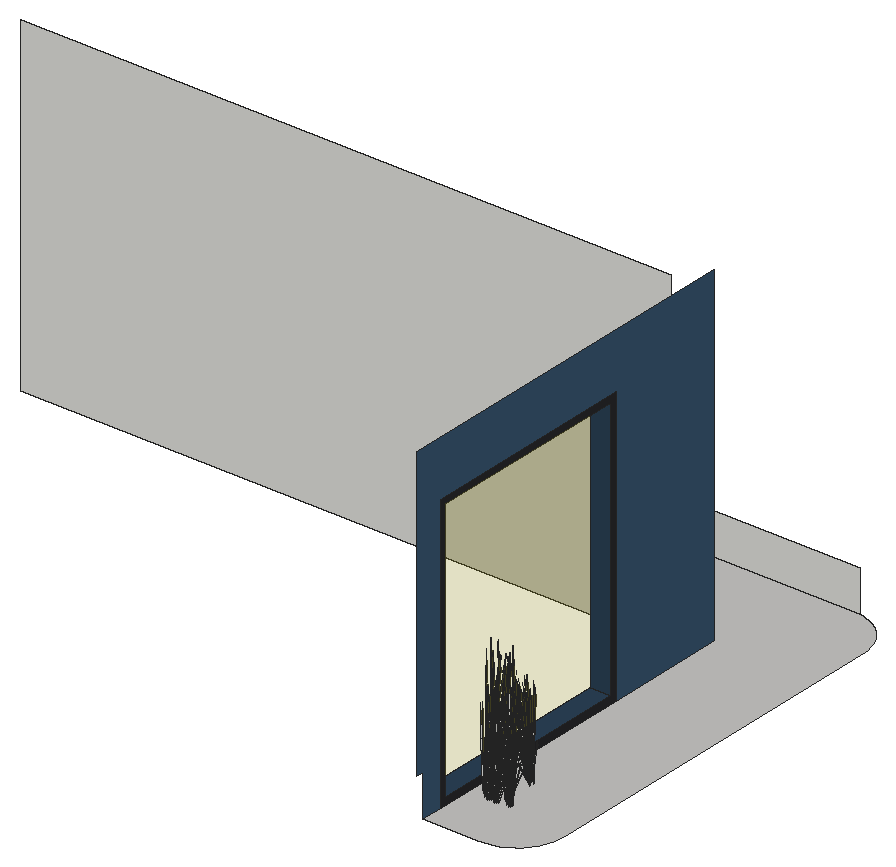
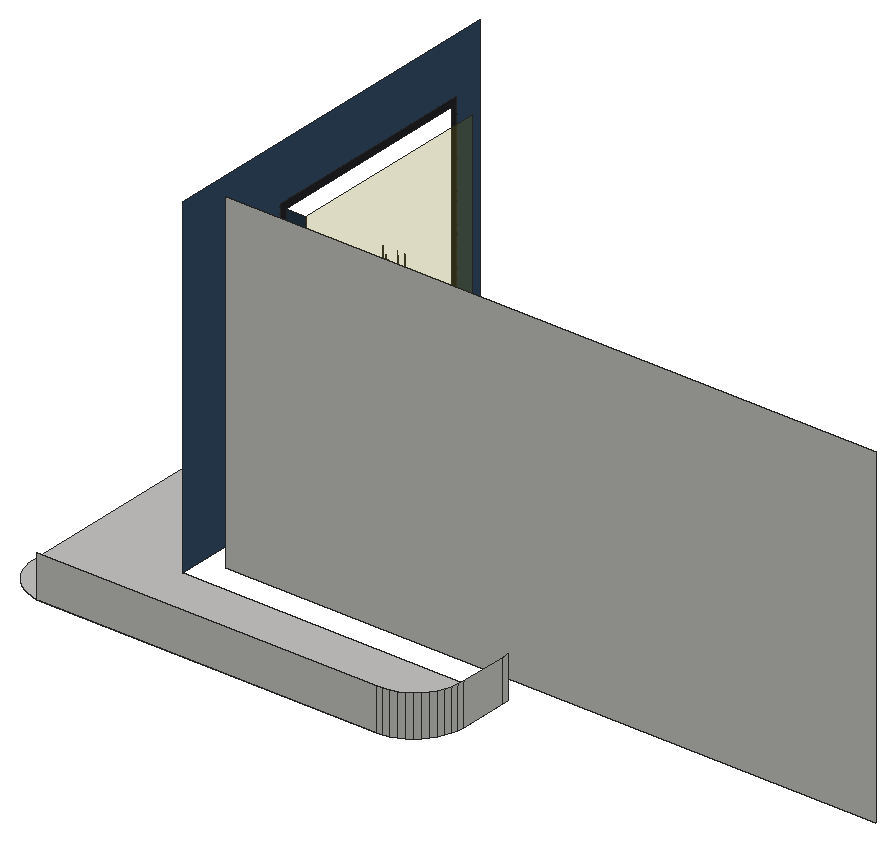
# SketchUp Ruby script. Lengths in inches.
U = 1.inch
M = Sketchup.active_model
def pt(a) = Geom::Point3d.new(a.map { |v| v * U })
def face(e, loops, mat)
  f = e.add_face(loops[0].map { |a| pt(a) })
  loops[1..].each { |l| e.add_face(l.map { |a| pt(a) }).erase! }
  f.material = f.back_material = mat if mat
  f
end
# faces: each face lists its corners as indices into pts; further lists are holes
def faces(e, pts, list, mat = nil) = list.each { |f| face(e, (f[0].is_a?(Array) ? f : [f]).map { |l| l.map { |i| pts[i] } }, mat) }
# xy, xz, yz: faces in a plane at the given z, y or x. An outline is a flat list of corners, or four numbers for a rectangle; further outlines are holes
def ring(l) = l.size == 4 ? [[l[0], l[1]], [l[2], l[1]], [l[2], l[3]], [l[0], l[3]]] : l.each_slice(2).to_a
def flat(e, list, mat, &to3) = list.each { |f| face(e, (f[0].is_a?(Array) ? f : [f]).map { |l| ring(l).map { |u, v| to3.(u, v) } }, mat) }
def xy(e, z, list, mat = nil) = flat(e, list, mat) { |x, y| [x, y, z] }
def xz(e, y, list, mat = nil) = flat(e, list, mat) { |x, z| [x, y, z] }
def yz(e, x, list, mat = nil) = flat(e, list, mat) { |y, z| [x, y, z] }
def lines(e, pts, list) = list.each { |a, b| e.add_line(pt(pts[a]), pt(pts[b])) }
# prism: a flat outline (further loops are holes) pulled along v
def prism(e, loops, v, mat = nil)
  f = face(e, loops, mat); d = Geom::Vector3d.new(v.map { |x| x * U })
  f.pushpull(f.normal.samedirection?(d) ? d.length : -d.length)
end
def box(e, o, s, mat = nil) = prism(e, [[o, [o[0] + s[0], o[1], o[2]], [o[0] + s[0], o[1] + s[1], o[2]], [o[0], o[1] + s[1], o[2]]]], [0, 0, s[2]], mat)
def at(x, y, z, deg = 0) = Geom::Transformation.translation(pt([x, y, z])) * Geom::Transformation.rotation(ORIGIN, Z_AXIS, deg.degrees)
def axes(o, x, y, z) = Geom::Transformation.new([*x, 0, *y, 0, *z, 0, *pt(o).to_a, 1])
def part(name) = M.definitions.add(name)
# library, detail: a bought-in or finely detailed component or shape, given as its bounding box
def library(name, o, s) = part(name).tap { |d| box(d.entities, o, s) }
def detail(e, o, s) = box(e.add_group.entities, o, s)
def put(e, d, t, mat = nil) = e.add_instance(d, t).tap { |i| i.material = mat if mat }
def group(e, t, mat = nil) = e.add_group.tap { |g| g.transformation = t; g.material = mat if mat }.entities
root = M.entities
M.materials.add("Carpet_01_1K").color = [196, 195, 193]
M.materials.add("Carpet_04_1K").color = [56, 85, 112]
M.materials.add("Carpet_04_1K1").color = [43, 65, 85]
M.materials.add("Glass_Basic_01").color = [186, 175, 28]
M.materials["Glass_Basic_01"].alpha = 0.25
M.materials.add("LightPink_Translucent").color = [144, 107, 117]
M.materials["LightPink_Translucent"].alpha = 0.75
M.materials.add("ThomThom - Buttons2").color = [40, 40, 43]
c1 = part("blade")
p = [[2.15,0.21,22],[0,0.17,0],[0.09,0.45,0],[2.18,0.31,22],[2.29,0.31,22],[0.38,0.45,0],
  [2.48,0.24,33],[2.49,0.24,33],[2.48,0.22,33]]
faces(c1.entities,p,[[0,1,2,3],[4,5,2,3],[6,3,4,7],[8,0,3,6]])
c2 = part("seeds")
p = [[0.3,-0.1,1.38],[-0.01,-0.03,1.59],[-0.01,-0.03,0.03],[0.14,-0.07,-0.07],[0.29,-0.03,3],[0.15,0.01,3.11]]
faces(c2.entities,p,[[0,1,2,3],[1,0,4,5]],"LightPink_Translucent")
c3 = part("blade with seeds")
put(c3.entities,c1,at(0,0,0))
put(c3.entities,c2,axes([2.4,0.25,30.99],[1.5799,-0.05474,1.17369],[-0.12525,1.92788,0.29478],[-0.07173,-0.02425,1.56792]))
xy(root,618,[[330.57,640.9,354.57,640.9,357.32,641.08,360.01,641.62,362.61,642.5,365.07,643.71,367.36,645.24,369.42,647.05,371.24,649.12,372.76,651.4,373.98,653.86,374.86,656.47,375.4,659.16,375.57,661.9,375.57,822.84,375.39,825.68,374.85,828.375,373.97,830.97,372.76,833.4375,371.23,835.72,369.42,837.79,367.36,839.6,365.07,841.12,362.61,842.34,360.01,843.22,357.59,843.7,210.57,843.7,207.83,843.52,205.14,842.99,202.54,842.1,200.07,840.89,197.79,839.36,195.73,837.55,193.91,835.48,192.39,833.2,191.17,830.74,190.29,828.14,189.75,825.44,189.57,822.7,189.57,798.7,330.57,798.7]],"Carpet_01_1K")
xy(root,621,[[321.57,652.9,330.57,742.9]],"Carpet_04_1K1")
xz(root,742.9,[[321.57,621,330.57,735]],"Carpet_04_1K1")
xz(root,786.64,[[39.57,618,321.57,762]])
xz(root,843.7,[[210.57,618,357.59,636]])
yz(root,189.57,[[798.7,618,801.7,636],[801.7,618,822.7,636]])
yz(root,321.57,[[652.9,621,742.9,735]],"Glass_Basic_01")
yz(root,330.57,[[640.9,618,649.9,618,649.9,738,745.9,738,745.9,618,798.7,618,798.7,762,637.9,762,637.9,636,640.9,636]],"Carpet_04_1K")
yz(root,330.57,[[[649.9,618,745.9,738],[652.9,621,742.9,735]]],"ThomThom - Buttons2")
p = [[189.57,822.7,618],[189.75,825.44,618],[189.75,825.44,636],[189.57,822.7,636],[190.29,828.14,618],[190.29,828.14,636],
  [191.17,830.74,618],[191.17,830.74,636],[192.39,833.2,618],[192.39,833.2,636],[193.91,835.48,618],[193.91,835.48,636],
  [195.73,837.55,618],[195.73,837.55,636],[197.79,839.36,618],[197.79,839.36,636],[200.07,840.89,618],[200.07,840.89,636],
  [202.54,842.1,618],[202.54,842.1,636],[205.14,842.99,618],[205.14,842.99,636],[207.83,843.52,618],[207.83,843.52,636],
  [210.57,843.7,618],[210.57,843.7,636]]
faces(root,p,[[0,1,2,3],[1,4,5,2],[4,6,7,5],[6,8,9,7],[8,10,11,9],[10,12,13,11],[12,14,15,13],[14,16,17,15],
  [16,18,19,17],[18,20,21,19],[20,22,23,21],[22,24,25,23]])
put(root,c3,axes([342.2,662.9,622.53],[-0.30722,0.06665,-0.35414],[-0.08112,-0.381,0.4572],[-0.08804,0.10234,0.87481]))
put(root,c3,axes([341.27,662.46,620.21],[-0.17124,0.42022,-0.44739],[-0.35581,-0.20224,0.21531],[0,0.09687,1.43643]))
put(root,c3,axes([339.09,662.92,622.53],[-0.30722,0.06665,-0.35414],[-0.08112,-0.381,0.4572],[-0.08804,0.10234,0.87481]))
put(root,c3,axes([350.55,662.74,620.67],[0.04113,0.53214,-0.29095],[-0.42835,0.03218,-0.50002],[-0.07543,0.07088,1.59708]))
put(root,c3,axes([345.11,663.43,622.73],[-0.26024,0.30729,0.48003],[-0.22444,-0.32634,0.3958],[0.1221,0.05668,0.9933]))
put(root,c3,axes([342,663.45,622.73],[-0.26024,0.30729,0.48003],[-0.22444,-0.32634,0.3958],[0.1221,0.05668,0.9933]))
put(root,c3,axes([350.7,662.54,620.21],[-0.17124,0.42022,-0.44739],[-0.35581,-0.20224,0.21531],[0,0.09687,1.43643]))
put(root,c3,axes([348.53,663,622.53],[-0.30722,0.06665,-0.35414],[-0.08112,-0.381,0.4572],[-0.08804,0.10234,0.87481]))
put(root,c3,axes([341.76,663.76,623.65],[0.31145,0.12449,-0.06488],[-0.0958,0.38314,-0.29416],[-0.05094,0.05817,0.97024]))
put(root,c3,axes([343.97,663.05,620.06],[-0.23773,0.35053,-0.62353],[-0.29532,-0.31785,-0.16365],[-0.09526,0.08744,1.37633]))
put(root,c3,axes([338.64,663.78,623.65],[0.31145,0.12449,-0.06488],[-0.0958,0.38314,-0.29416],[-0.05094,0.05817,0.97024]))
put(root,c3,axes([340.85,663.07,620.06],[-0.23773,0.35053,-0.62353],[-0.29532,-0.31785,-0.16365],[-0.09526,0.08744,1.37633]))
put(root,c3,axes([344.28,663.78,623.05],[-0.05451,-0.37564,0.35414],[0.31161,-0.09919,-0.4572],[0.0837,0.10765,0.87481]))
put(root,c3,axes([348.08,663.86,623.65],[0.31145,0.12449,-0.06488],[-0.0958,0.38314,-0.29416],[-0.05094,0.05817,0.97024]))
put(root,c3,axes([350.29,663.15,620.06],[-0.23773,0.35053,-0.62353],[-0.29532,-0.31785,-0.16365],[-0.09526,0.08744,1.37633]))
put(root,c3,axes([341.17,663.8,623.05],[-0.05451,-0.37564,0.35414],[0.31161,-0.09919,-0.4572],[0.0837,0.10765,0.87481]))
put(root,c3,axes([344.39,663.64,620.33],[0.44186,0.15158,0.30756],[-0.11054,0.54181,-0.36492],[-0.07313,0.06781,1.64885]))
put(root,c3,axes([344.36,664.01,620.02],[-0.33032,0.23318,-0.49651],[-0.19744,-0.41812,0],[-0.07523,0.05311,1.57504]))
put(root,c3,axes([341.27,663.66,620.33],[0.44186,0.15158,0.30756],[-0.11054,0.54181,-0.36492],[-0.07313,0.06781,1.64885]))
put(root,c3,axes([345.45,662.625,620.02],[0,0.46636,-0.49651],[-0.39487,0,0],[0,0.10622,1.57504]))
put(root,c3,axes([341.24,664.03,620.02],[-0.33032,0.23318,-0.49651],[-0.19744,-0.41812,0],[-0.07523,0.05311,1.57504]))
put(root,c3,axes([342.34,662.65,620.02],[0,0.46636,-0.49651],[-0.39487,0,0],[0,0.10622,1.57504]))
put(root,c3,axes([344.47,662.68,621.875],[-0.1311,-0.08035,1.71376],[0.27131,-0.33708,0.13857],[0.16909,0.15206,0.73262]))
put(root,c3,axes([341.35,662.7,621.875],[-0.1311,-0.08035,1.71376],[0.27131,-0.33708,0.13857],[0.16909,0.15206,0.73262]))
put(root,c3,axes([350.71,663.74,620.33],[0.44186,0.15158,0.30756],[-0.11054,0.54181,-0.36492],[-0.07313,0.06781,1.64885]))
put(root,c3,axes([344.49,661.62,622.47],[-0.30498,-0.24231,1.38283],[0.32203,-0.37727,0.59665],[0.0984,0.22736,1.33663]))
put(root,c3,axes([350.68,664.11,620.02],[-0.33032,0.23318,-0.49651],[-0.19744,-0.41812,0],[-0.07523,0.05311,1.57504]))
put(root,c3,axes([341.38,661.64,622.47],[-0.30498,-0.24231,1.38283],[0.32203,-0.37727,0.59665],[0.0984,0.22736,1.33663]))
put(root,c3,axes([342.29,662.64,623.03],[0.32648,0.25715,-0.1216],[-0.18809,0.3724,-0.67495],[-0.09224,0.12945,1.02557]))
put(root,c3,axes([339.18,662.66,623.03],[0.32648,0.25715,-0.1216],[-0.18809,0.3724,-0.67495],[-0.09224,0.12945,1.02557]))
put(root,c3,axes([344.95,663.59,620.77],[-0.19872,-0.13409,1.1486],[0.2566,-0.13625,0.84392],[0.06921,0.11541,0.25299]))
put(root,c3,axes([341.84,663.62,620.77],[-0.19872,-0.13409,1.1486],[0.2566,-0.13625,0.84392],[0.06921,0.11541,0.25299]))
put(root,c3,axes([344.25,663.98,623.03],[0.21031,-0.39918,-0.1216],[0.30457,0.22997,-0.67495],[0.10587,0.11278,1.02557]))
put(root,c3,axes([341.14,664,623.03],[0.21031,-0.39918,-0.1216],[0.30457,0.22997,-0.67495],[0.10587,0.11278,1.02557]))
put(root,c3,axes([348.62,662.74,623.03],[0.32648,0.25715,-0.1216],[-0.18809,0.3724,-0.67495],[-0.09224,0.12945,1.02557]))
put(root,c3,axes([342.73,662.53,621.875],[0.08815,-0.14329,1.71376],[0.22258,0.38678,0.13857],[-0.15267,0.17614,0.73262]))
put(root,c3,axes([339.62,662.55,621.875],[0.08815,-0.14329,1.71376],[0.22258,0.38678,0.13857],[-0.15267,0.17614,0.73262]))
put(root,c3,axes([342.46,662.95,622.68],[0.09067,0.42583,-0.51099],[-0.34336,0.07449,-0.3958],[-0.0984,0.11438,0.97773]))
put(root,c3,axes([339.34,662.97,622.68],[0.09067,0.42583,-0.51099],[-0.34336,0.07449,-0.3958],[-0.0984,0.11438,0.97773]))
put(root,c3,axes([349.06,662.63,621.875],[0.08815,-0.14329,1.71376],[0.22258,0.38678,0.13857],[-0.15267,0.17614,0.73262]))
put(root,c3,axes([342.87,663.4375,623.05],[0.23881,-0.24554,0.35414],[0.22606,0.28036,-0.4572],[-0.0344,0.14245,0.87481]))
put(root,c3,axes([344.66,663.93,620.375],[0.22066,0.46731,0],[-0.36918,0.26061,-0.51607],[-0.08408,0.05936,1.63711]))
put(root,c3,axes([339.75,663.46,623.05],[0.23881,-0.24554,0.35414],[0.22606,0.28036,-0.4572],[-0.0344,0.14245,0.87481]))
put(root,c3,axes([348.78,663.05,622.68],[0.09067,0.42583,-0.51099],[-0.34336,0.07449,-0.3958],[-0.0984,0.11438,0.97773]))
put(root,c3,axes([341.54,663.96,620.375],[0.22066,0.46731,0],[-0.36918,0.26061,-0.51607],[-0.08408,0.05936,1.63711]))
put(root,c3,axes([343.98,664.31,622.71],[0.00104,-0.05646,1.77383],[0.30246,-0.2491,-0.16761],[0.10506,0.08891,0.31391]))
put(root,c3,axes([340.87,664.33,622.71],[0.00104,-0.05646,1.77383],[0.30246,-0.2491,-0.16761],[0.10506,0.08891,0.31391]))
put(root,c3,axes([345.01,664.09,619.49],[0.02571,-0.06733,1.76342],[0.32373,-0.19829,-0.26939],[0.09815,0.10263,0.30037]))
put(root,c3,axes([349.19,663.54,623.05],[0.23881,-0.24554,0.35414],[0.22606,0.28036,-0.4572],[-0.0344,0.14245,0.87481]))
put(root,c3,axes([344.47,662.08,620.84],[-0.00964,-0.43909,1.41272],[0.43635,0.11382,0.59816],[-0.1032,0.24027,1.3335]))
put(root,c3,axes([344.58,662.5625,620.09],[0.12941,0.42699,-0.69212],[-0.37279,0.15378,-0.18165],[0.0143,0.14459,1.52773]))
put(root,c3,axes([341.89,664.11,619.49],[0.02571,-0.06733,1.76342],[0.32373,-0.19829,-0.26939],[0.09815,0.10263,0.30037]))
put(root,c3,axes([342.65,663.66,622.73],[-0.29004,-0.02173,0.0643],[0.00795,-0.32812,0.50621],[-0.03035,0.12569,0.77189]))
put(root,c3,axes([350.98,664.03,620.375],[0.22066,0.46731,0],[-0.36918,0.26061,-0.51607],[-0.08408,0.05936,1.63711]))
put(root,c3,axes([341.35,662.11,620.84],[-0.00964,-0.43909,1.41272],[0.43635,0.11382,0.59816],[-0.1032,0.24027,1.3335]))
put(root,c3,axes([341.47,662.58,620.09],[0.12941,0.42699,-0.69212],[-0.37279,0.15378,-0.18165],[0.0143,0.14459,1.52773]))
put(root,c3,axes([339.54,663.68,622.73],[-0.29004,-0.02173,0.0643],[0.00795,-0.32812,0.50621],[-0.03035,0.12569,0.77189]))
put(root,c3,axes([342.04,664.03,619.49],[0.04734,0.04659,1.76342],[0.08027,0.4317,-0.26939],[-0.10492,0.09206,0.30037]))
put(root,c3,axes([342.74,663.69,622.73],[-0.25132,-0.3182,0.48003],[0.2669,-0.27442,0.3958],[-0.04636,0.14929,0.9933]))
put(root,c3,axes([338.92,664.06,619.49],[0.04734,0.04659,1.76342],[0.08027,0.4317,-0.26939],[-0.10492,0.09206,0.30037]))
put(root,c3,axes([344.5,663.78,622.68],[0.34827,-0.11086,-0.51099],[0.06092,0.41983,-0.3958],[0.09354,0.12031,0.97773]))
put(root,c3,axes([339.63,663.71,622.73],[-0.25132,-0.3182,0.48003],[0.2669,-0.27442,0.3958],[-0.04636,0.14929,0.9933]))
put(root,c3,axes([341.39,663.8,622.68],[0.34827,-0.11086,-0.51099],[0.06092,0.41983,-0.3958],[0.09354,0.12031,0.97773]))
put(root,c3,axes([350.79,662.18,620.84],[-0.00964,-0.43909,1.41272],[0.43635,0.11382,0.59816],[-0.1032,0.24027,1.3335]))
put(root,c3,axes([348.98,663.76,622.73],[-0.29004,-0.02173,0.0643],[0.00795,-0.32812,0.50621],[-0.03035,0.12569,0.77189]))
put(root,c3,axes([348.36,664.13,619.49],[0.04734,0.04659,1.76342],[0.08027,0.4317,-0.26939],[-0.10492,0.09206,0.30037]))
put(root,c3,axes([343.54,663.84,623.05],[0.1064,-0.35863,0.35414],[0.31043,0.1046,-0.4572],[0.02846,0.14439,0.87481]))
put(root,c3,axes([349.07,663.79,622.73],[-0.25132,-0.3182,0.48003],[0.2669,-0.27442,0.3958],[-0.04636,0.14929,0.9933]))
put(root,c3,axes([340.42,663.86,623.05],[0.1064,-0.35863,0.35414],[0.31043,0.1046,-0.4572],[0.02846,0.14439,0.87481]))
put(root,c3,axes([349.86,663.94,623.05],[0.1064,-0.35863,0.35414],[0.31043,0.1046,-0.4572],[0.02846,0.14439,0.87481]))
put(root,c3,axes([344.98,664.2,620.67],[-0.22633,-0.01463,1.0506],[0.14947,-0.31064,0.58006],[0.08941,0.11036,0.8241]))
put(root,c3,axes([341.87,664.23,620.67],[-0.22633,-0.01463,1.0506],[0.14947,-0.31064,0.58006],[0.08941,0.11036,0.8241]))
put(root,c3,axes([344.33,664.12,622.73],[-0.16041,0.29625,0.0643],[-0.22843,-0.17248,0.50621],[0.07385,0.09498,0.77189]))
put(root,c3,axes([341.22,664.14,622.73],[-0.16041,0.29625,0.0643],[-0.22843,-0.17248,0.50621],[0.07385,0.09498,0.77189]))
put(root,c3,axes([343.96,665.12,623.65],[0.2439,-0.26754,-0.06488],[0.22348,0.29302,-0.29416],[0.01573,0.08303,0.97024]))
put(root,c3,axes([340.84,665.14,623.65],[0.2439,-0.26754,-0.06488],[0.22348,0.29302,-0.29416],[0.01573,0.08303,0.97024]))
put(root,c3,axes([344.4,664.04,622.73],[-0.35104,0.10702,0.48003],[-0.06092,-0.41983,0.3958],[0.08256,0.12373,0.9933]))
put(root,c3,axes([341.29,664.0625,622.73],[-0.35104,0.10702,0.48003],[-0.06092,-0.41983,0.3958],[0.08256,0.12373,0.9933]))
put(root,c3,axes([350.28,665.22,623.65],[0.2439,-0.26754,-0.06488],[0.22348,0.29302,-0.29416],[0.01573,0.08303,0.97024]))
put(root,c3,axes([342.67,662.88,621.875],[0.06572,-0.16029,1.71376],[0.27569,0.33172,0.13857],[-0.12437,0.20675,0.73262]))
put(root,c3,axes([339.55,662.9,621.875],[0.06572,-0.16029,1.71376],[0.27569,0.33172,0.13857],[-0.12437,0.20675,0.73262]))
put(root,c3,axes([344.25,663.45,620.59],[0.00623,-0.15459,1.43002],[0.29764,-0.17268,-0.30754],[0.09188,0.18503,0.61141]))
put(root,c3,axes([348.99,662.98,621.875],[0.06572,-0.16029,1.71376],[0.27569,0.33172,0.13857],[-0.12437,0.20675,0.73262]))
put(root,c3,axes([341.13,663.47,620.59],[0.00623,-0.15459,1.43002],[0.29764,-0.17268,-0.30754],[0.09188,0.18503,0.61141]))
put(root,c3,axes([343.44,664.17,622.73],[-0.26007,0.1585,0.0643],[-0.12729,-0.28902,0.50621],[0.02512,0.1274,0.77189]))
put(root,c3,axes([342.74,663.79,622.53],[-0.23881,0.24554,-0.35414],[-0.22606,-0.28036,0.4572],[-0.0344,0.14245,0.87481]))
put(root,c3,axes([341.92,663.71,622.72],[-0.00877,0.09229,1.74944],[0.24897,0.32105,-0.27667],[-0.06518,0.15182,0.14031]))
put(root,c3,axes([340.33,664.1875,622.73],[-0.26007,0.1585,0.0643],[-0.12729,-0.28902,0.50621],[0.02512,0.1274,0.77189]))
put(root,c3,axes([342.72,663.5,623.4],[0.3879,0.02311,-0.13498],[-0.0106,0.43749,-0.74919],[-0.02694,0.1685,1.13838]))
put(root,c3,axes([339.63,663.81,622.53],[-0.23881,0.24554,-0.35414],[-0.22606,-0.28036,0.4572],[-0.0344,0.14245,0.87481]))
put(root,c3,axes([338.81,663.73,622.72],[-0.00877,0.09229,1.74944],[0.24897,0.32105,-0.27667],[-0.06518,0.15182,0.14031]))
put(root,c3,axes([343.43,663.99,623.03],[0.34538,-0.21713,-0.1216],[0.16972,0.38536,-0.67495],[0.04557,0.16239,1.02557]))
put(root,c3,axes([339.6,663.53,623.4],[0.3879,0.02311,-0.13498],[-0.0106,0.43749,-0.74919],[-0.02694,0.1685,1.13838]))
put(root,c3,axes([340.32,664.01,623.03],[0.34538,-0.21713,-0.1216],[0.16972,0.38536,-0.67495],[0.04557,0.16239,1.02557]))
put(root,c3,axes([343.53,664.14,623.0625],[-0.34777,-0.12192,0.53283],[0.11892,-0.40083,0.43934],[0.0209,0.15763,1.10256]))
put(root,c3,axes([349.77,664.27,622.73],[-0.26007,0.1585,0.0643],[-0.12729,-0.28902,0.50621],[0.02512,0.1274,0.77189]))
put(root,c3,axes([340.42,664.16,623.0625],[-0.34777,-0.12192,0.53283],[0.11892,-0.40083,0.43934],[0.0209,0.15763,1.10256]))
put(root,c3,axes([349.07,663.89,622.53],[-0.23881,0.24554,-0.35414],[-0.22606,-0.28036,0.4572],[-0.0344,0.14245,0.87481]))
put(root,c3,axes([348.24,663.8125,622.72],[-0.00877,0.09229,1.74944],[0.24897,0.32105,-0.27667],[-0.06518,0.15182,0.14031]))
put(root,c3,axes([342.9,664.74,620.77],[-0.00913,-0.2773,1.1486],[0.22824,0.19778,0.84392],[-0.04489,0.13217,0.25299]))
put(root,c3,axes([349.04,663.6,623.4],[0.3879,0.02311,-0.13498],[-0.0106,0.43749,-0.74919],[-0.02694,0.1685,1.13838]))
put(root,c3,axes([339.78,664.76,620.77],[-0.00913,-0.2773,1.1486],[0.22824,0.19778,0.84392],[-0.04489,0.13217,0.25299]))
put(root,c3,axes([349.86,664.24,623.0625],[-0.34777,-0.12192,0.53283],[0.11892,-0.40083,0.43934],[0.0209,0.15763,1.10256]))
put(root,c3,axes([349.22,664.84,620.77],[-0.00913,-0.2773,1.1486],[0.22824,0.19778,0.84392],[-0.04489,0.13217,0.25299]))
put(root,c3,axes([343.5,664.08,619.49],[0.05712,-0.02538,1.76342],[0.34359,0.13968,-0.26939],[0.01005,0.15742,0.30037]))
put(root,c3,axes([340.38,664.1,619.49],[0.05712,-0.02538,1.76342],[0.34359,0.13968,-0.26939],[0.01005,0.15742,0.30037]))
put(root,c3,axes([349.82,664.18,619.49],[0.05712,-0.02538,1.76342],[0.34359,0.13968,-0.26939],[0.01005,0.15742,0.30037]))
put(root,c3,axes([342.98,663.67,623],[0.25266,0.31335,-0.5672],[-0.2669,0.27442,-0.43934],[-0.03844,0.15921,1.08528]))
put(root,c3,axes([339.87,663.69,623],[0.25266,0.31335,-0.5672],[-0.2669,0.27442,-0.43934],[-0.03844,0.15921,1.08528]))
put(root,c3,axes([342.71,664.14,620.82],[0.32063,-0.08258,0.06507],[0.07371,0.33271,-0.86304],[-0.02033,0.16842,0.7736]))
put(root,c3,axes([343.73,663.97,622.68],[0.34695,0.11691,-0.51099],[-0.11892,0.40083,-0.3958],[0.03181,0.16138,0.97773]))
put(root,c3,axes([343.93,663.15,621.875],[-0.08068,-0.14973,1.71376],[0.3728,-0.12606,0.13857],[0.08426,0.23506,0.73262]))
put(root,c3,axes([349.31,663.77,623],[0.25266,0.31335,-0.5672],[-0.2669,0.27442,-0.43934],[-0.03844,0.15921,1.08528]))
put(root,c3,axes([339.59,664.16,620.82],[0.32063,-0.08258,0.06507],[0.07371,0.33271,-0.86304],[-0.02033,0.16842,0.7736]))
put(root,c3,axes([340.62,663.99,622.68],[0.34695,0.11691,-0.51099],[-0.11892,0.40083,-0.3958],[0.03181,0.16138,0.97773]))
put(root,c3,axes([340.8125,663.17,621.875],[-0.08068,-0.14973,1.71376],[0.3728,-0.12606,0.13857],[0.08426,0.23506,0.73262]))
put(root,c3,axes([349.03,664.24,620.82],[0.32063,-0.08258,0.06507],[0.07371,0.33271,-0.86304],[-0.02033,0.16842,0.7736]))
put(root,c3,axes([343.57,664.22,622.53],[-0.1064,0.35863,-0.35414],[-0.31043,-0.1046,0.4572],[0.02846,0.14439,0.87481]))
put(root,c3,axes([340.46,664.24,622.53],[-0.1064,0.35863,-0.35414],[-0.31043,-0.1046,0.4572],[0.02846,0.14439,0.87481]))
put(root,c3,axes([349.9,664.32,622.53],[-0.1064,0.35863,-0.35414],[-0.31043,-0.1046,0.4572],[0.02846,0.14439,0.87481]))
put(root,c3,axes([342.9,663.53,623.34],[-0.00918,0.43138,-0.7886],[-0.38672,-0.02897,0.09517],[-0.04081,0.18275,1.11556]))
put(root,c3,axes([339.79,663.55,623.34],[-0.00918,0.43138,-0.7886],[-0.38672,-0.02897,0.09517],[-0.04081,0.18275,1.11556]))
put(root,c3,axes([341.89,664.66,622.71],[0.04004,-0.02816,1.77383],[0.33095,0.18728,-0.16761],[-0.00778,0.15594,0.31391]))
put(root,c3,axes([338.78,664.68,622.71],[0.04004,-0.02816,1.77383],[0.33095,0.18728,-0.16761],[-0.00778,0.15594,0.31391]))
put(root,c3,axes([349.23,663.625,623.34],[-0.00918,0.43138,-0.7886],[-0.38672,-0.02897,0.09517],[-0.04081,0.18275,1.11556]))
put(root,c3,axes([348.22,664.76,622.71],[0.04004,-0.02816,1.77383],[0.33095,0.18728,-0.16761],[-0.00778,0.15594,0.31391]))
put(root,c3,axes([343.27,663.22,621.875],[-0.00864,-0.17899,1.71376],[0.37441,0.11874,0.13857],[-0.02316,0.25508,0.73262]))
put(root,c3,axes([340.15,663.24,621.875],[-0.00864,-0.17899,1.71376],[0.37441,0.11874,0.13857],[-0.02316,0.25508,0.73262]))
put(root,c3,axes([349.59,663.32,621.875],[-0.00864,-0.17899,1.71376],[0.37441,0.11874,0.13857],[-0.02316,0.25508,0.73262]))
put(root,c3,axes([352.69,670.34,627.46],[0.1311,0.08035,1.71376],[-0.27131,0.33708,0.13857],[-0.16909,-0.15206,0.73262]))
put(root,c3,axes([343.6,663.9,622.98],[0.16845,0.3792,-0.71045],[-0.34676,0.21133,0.08574],[0.03939,0.18322,1.00501]))
put(root,c3,axes([340.49,663.92,622.98],[0.16845,0.3792,-0.71045],[-0.34676,0.21133,0.08574],[0.03939,0.18322,1.00501]))
put(root,c3,axes([349.93,664,622.98],[0.16845,0.3792,-0.71045],[-0.34676,0.21133,0.08574],[0.03939,0.18322,1.00501]))
put(root,c3,axes([342.63,664.49,620.59],[0.11138,-0.07357,1.43002],[0.27499,0.22183,-0.30754],[-0.08185,0.19194,0.61141]))
put(root,c3,axes([339.51,664.51,620.59],[0.11138,-0.07357,1.43002],[0.27499,0.22183,-0.30754],[-0.08185,0.19194,0.61141]))
put(root,c3,axes([343.35,664.85,622.72],[0.04474,0.0751,1.74944],[0.36104,0.0295,-0.27667],[0.03631,0.16562,0.14031]))
put(root,c3,axes([340.24,664.875,622.72],[0.04474,0.0751,1.74944],[0.36104,0.0295,-0.27667],[0.03631,0.16562,0.14031]))
put(root,c3,axes([348.95,664.59,620.59],[0.11138,-0.07357,1.43002],[0.27499,0.22183,-0.30754],[-0.08185,0.19194,0.61141]))
put(root,c3,axes([349.68,664.95,622.72],[0.04474,0.0751,1.74944],[0.36104,0.0295,-0.27667],[0.03631,0.16562,0.14031]))
put(root,c3,axes([352.66,669.6,628.3],[-0.07594,-0.00329,1.74944],[-0.24177,0.32918,-0.27667],[-0.129,-0.06726,0.14031]))
put(root,c3,axes([342.77,664.13,621.36],[0.00775,-0.24075,1.54345],[0.34877,0.12716,0.21329],[-0.03022,0.25658,0.72882]))
put(root,c3,axes([339.66,664.16,621.36],[0.00775,-0.24075,1.54345],[0.34877,0.12716,0.21329],[-0.03022,0.25658,0.72882]))
put(root,c3,axes([349.1,664.23,621.36],[0.00775,-0.24075,1.54345],[0.34877,0.12716,0.21329],[-0.03022,0.25658,0.72882]))
put(root,c3,axes([352.61,670.34,628.68],[0.29147,-0.34417,0.53763],[0.25138,0.3655,0.4433],[-0.13675,-0.06349,1.11249]))
put(root,c3,axes([352.74,670.34,628.32],[0.01777,-0.35463,0.0643],[0.26836,0.00972,0.50621],[-0.1028,-0.03711,0.77189]))
put(root,c3,axes([352.64,670.45,628.12],[-0.20082,-0.29199,-0.35414],[0.2293,-0.2764,0.4572],[-0.1165,-0.04206,0.87481]))
put(root,c3,axes([352.57,670.76,626.18],[0.06891,0.12984,1.43002],[-0.15879,0.35293,-0.30754],[-0.16304,-0.08436,0.61141]))
put(root,c3,axes([352.85,670.65,628.57],[-0.35281,-0.01123,-0.71045],[0.0237,-0.47284,0.08574],[-0.14947,-0.0499,1.00501]))
put(root,c3,axes([352.37,669.88,628.3],[0.02617,0.04654,1.77383],[-0.12614,0.41836,-0.16761],[-0.12775,0.00303,0.31391]))
put(root,c3,axes([352.73,670.74,628.27],[-0.25628,0.30892,-0.51099],[-0.22444,-0.32634,-0.3958],[-0.13021,-0.047,0.97773]))
put(root,c3,axes([352.16,671.15,626.35],[0.22533,-0.03337,1.1486],[-0.14293,0.29403,0.84392],[-0.11135,-0.04411,0.25299]))
put(root,c3,axes([352.87,670.42,628.62],[-0.0189,0.47427,-0.1216],[-0.35781,-0.01296,-0.67495],[-0.13781,-0.03295,1.02557]))
put(root,c3,axes([352.41,671.07,627.46],[0.14639,-0.01056,1.71376],[-0.09712,0.45778,0.13857],[-0.20862,-0.02831,0.73262]))
put(root,c3,axes([352.35,671.42,628.32],[0.09971,-0.42522,0.48003],[0.32782,0.1454,0.3958],[-0.12892,0.02555,0.9933]))
put(root,c3,axes([352.33,671.31,628.32],[-0.12963,-0.31798,0.0643],[0.23638,-0.15564,0.50621],[-0.1042,0.03071,0.77189]))
put(root,c3,axes([352.32,671.63,625.08],[0.00895,0.0735,1.76342],[-0.18044,0.38382,-0.26939],[-0.12817,-0.01935,0.30037]))
put(root,c3,axes([352.28,671.47,628.12],[-0.29332,-0.1301,-0.35414],[0.08555,-0.37955,0.4572],[-0.11809,0.0348,0.87481]))
put(root,c3,axes([352.59,671.42,628.64],[0.29332,0.1301,0.35414],[-0.08555,0.37955,-0.4572],[-0.11809,0.0348,0.87481]))
put(root,c3,axes([353.18,671.4,626.93],[0.10032,-0.06746,1.77064],[0.0346,0.47103,0.13857],[-0.2173,0.0625,0.63284]))
put(root,c3,axes([352.1,671.72,628.3],[-0.05763,0.06055,1.74944],[0.0049,0.44239,-0.27667],[-0.13211,0.05753,0.14031]))
put(root,c3,axes([352.49,671.66,628.27],[-0.09562,0.42421,-0.51099],[-0.32782,-0.1454,-0.3958],[-0.13199,0.0389,0.97773]))
put(root,c3,axes([352.47,671.3,628.62],[0.17758,0.42229,-0.1216],[-0.31518,0.20752,-0.67495],[-0.13282,0.05572,1.02557]))
put(root,c3,axes([352.43,672.48,628.32],[-0.08753,-0.42921,0.48003],[0.34336,-0.07449,0.3958],[-0.1012,0.10094,0.9933]))
put(root,c3,axes([352.36,672.4,628.32],[-0.2423,-0.19613,0.0643],[0.14107,-0.2793,0.50621],[-0.07768,0.0903,0.77189]))
put(root,c3,axes([352.47,671.88,627.46],[0.12246,-0.09864,1.71376],[0.1031,0.45582,0.13857],[-0.19225,0.10302,0.73262]))
put(root,c3,axes([352.09,672.66,626.18],[0.12266,0.03828,1.43002],[0.07906,0.39104,-0.30754],[-0.16661,0.0732,0.61141]))
put(root,c3,axes([351.46,672.17,628.3],[0.04504,0.01251,1.77383],[0.13934,0.41205,-0.16761],[-0.0922,0.10815,0.31391]))
put(root,c3,axes([351.84,673.47,626.35],[0.14709,-0.21136,1.1486],[0.05804,0.3346,0.84392],[-0.1063,0.05991,0.25299]))
put(root,c3,axes([352.39,672.56,628.12],[-0.30722,0.06665,-0.35414],[-0.08112,-0.381,0.4572],[-0.08804,0.10234,0.87481]))
put(root,c3,axes([352.92,672.19,627.46],[0.08815,-0.14329,1.71376],[0.22258,0.38678,0.13857],[-0.15267,0.17614,0.73262]))
put(root,c3,axes([352.65,672.61,628.27],[0.09067,0.42583,-0.51099],[-0.34336,0.07449,-0.3958],[-0.0984,0.11438,0.97773]))
put(root,c3,axes([352.22,673.69,625.08],[0.04734,0.04659,1.76342],[0.08027,0.4317,-0.26939],[-0.10492,0.09206,0.30037]))
put(root,c3,axes([352.86,672.54,627.46],[0.06572,-0.16029,1.71376],[0.27569,0.33172,0.13857],[-0.12437,0.20675,0.73262]))
put(root,c3,axes([352.11,673.37,628.3],[-0.00877,0.09229,1.74944],[0.24897,0.32105,-0.27667],[-0.06518,0.15182,0.14031]))
